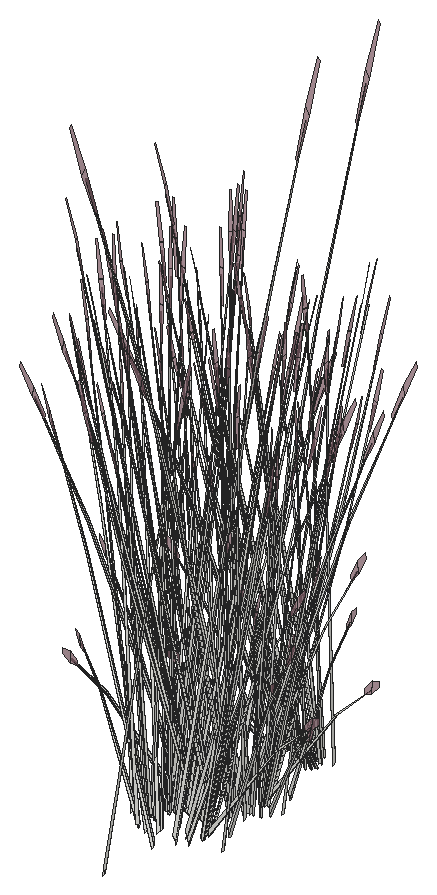
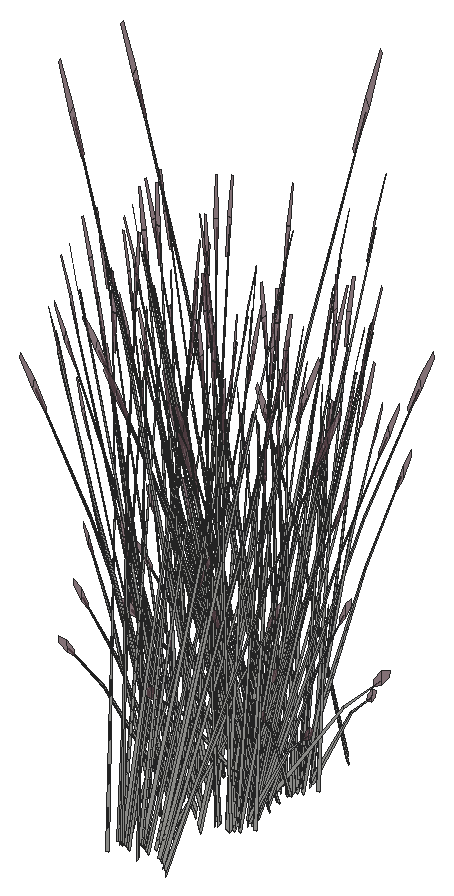
# SketchUp Ruby script. Lengths in inches.
U = 1.inch
M = Sketchup.active_model
def pt(a) = Geom::Point3d.new(a.map { |v| v * U })
def face(e, loops, mat)
  f = e.add_face(loops[0].map { |a| pt(a) })
  loops[1..].each { |l| e.add_face(l.map { |a| pt(a) }).erase! }
  f.material = f.back_material = mat if mat
  f
end
# faces: each face lists its corners as indices into pts; further lists are holes
def faces(e, pts, list, mat = nil) = list.each { |f| face(e, (f[0].is_a?(Array) ? f : [f]).map { |l| l.map { |i| pts[i] } }, mat) }
# xy, xz, yz: faces in a plane at the given z, y or x. An outline is a flat list of corners, or four numbers for a rectangle; further outlines are holes
def ring(l) = l.size == 4 ? [[l[0], l[1]], [l[2], l[1]], [l[2], l[3]], [l[0], l[3]]] : l.each_slice(2).to_a
def flat(e, list, mat, &to3) = list.each { |f| face(e, (f[0].is_a?(Array) ? f : [f]).map { |l| ring(l).map { |u, v| to3.(u, v) } }, mat) }
def xy(e, z, list, mat = nil) = flat(e, list, mat) { |x, y| [x, y, z] }
def xz(e, y, list, mat = nil) = flat(e, list, mat) { |x, z| [x, y, z] }
def yz(e, x, list, mat = nil) = flat(e, list, mat) { |y, z| [x, y, z] }
def lines(e, pts, list) = list.each { |a, b| e.add_line(pt(pts[a]), pt(pts[b])) }
# prism: a flat outline (further loops are holes) pulled along v
def prism(e, loops, v, mat = nil)
  f = face(e, loops, mat); d = Geom::Vector3d.new(v.map { |x| x * U })
  f.pushpull(f.normal.samedirection?(d) ? d.length : -d.length)
end
def box(e, o, s, mat = nil) = prism(e, [[o, [o[0] + s[0], o[1], o[2]], [o[0] + s[0], o[1] + s[1], o[2]], [o[0], o[1] + s[1], o[2]]]], [0, 0, s[2]], mat)
def at(x, y, z, deg = 0) = Geom::Transformation.translation(pt([x, y, z])) * Geom::Transformation.rotation(ORIGIN, Z_AXIS, deg.degrees)
def axes(o, x, y, z) = Geom::Transformation.new([*x, 0, *y, 0, *z, 0, *pt(o).to_a, 1])
def part(name) = M.definitions.add(name)
# library, detail: a bought-in or finely detailed component or shape, given as its bounding box
def library(name, o, s) = part(name).tap { |d| box(d.entities, o, s) }
def detail(e, o, s) = box(e.add_group.entities, o, s)
def put(e, d, t, mat = nil) = e.add_instance(d, t).tap { |i| i.material = mat if mat }
def group(e, t, mat = nil) = e.add_group.tap { |g| g.transformation = t; g.material = mat if mat }.entities
root = M.entities
M.materials.add("LightPink_Translucent").color = [144, 107, 117]
M.materials["LightPink_Translucent"].alpha = 0.75
c1 = part("blade")
p = [[2.15,0.21,22],[0,0.17,0],[0.09,0.45,0],[2.18,0.31,22],[2.29,0.31,22],[0.38,0.45,0],
  [2.48,0.24,33],[2.49,0.24,33],[2.48,0.22,33]]
faces(c1.entities,p,[[0,1,2,3],[4,5,2,3],[6,3,4,7],[8,0,3,6]])
c2 = part("seeds")
p = [[0.3,-0.1,1.38],[-0.01,-0.03,1.59],[-0.01,-0.03,0.03],[0.14,-0.07,-0.07],[0.29,-0.03,3],[0.15,0.01,3.11]]
faces(c2.entities,p,[[0,1,2,3],[1,0,4,5]],"LightPink_Translucent")
c3 = part("blade with seeds")
put(c3.entities,c1,at(0,0,0))
put(c3.entities,c2,axes([2.4,0.25,30.99],[1.5799,-0.05474,1.17369],[-0.12525,1.92788,0.29478],[-0.07173,-0.02425,1.56792]))
put(root,c3,axes([429.55,431.71,154.25],[-0.40102,0.2196,-0.10273],[-0.19707,-0.38974,-0.57019],[-0.05291,-0.16424,0.8664]))
put(root,c3,axes([430.38,432.21,154.25],[-0.45039,-0.02337,-0.10273],[0.01231,-0.44247,-0.57019],[0.03129,-0.17041,0.8664]))
put(root,c3,axes([427.89,424.64,152.84],[0.009,-0.24349,1.30391],[0.40497,0.12861,0.18019],[-0.03509,0.2595,0.61571]))
put(root,c3,axes([430.35,431.92,153.82],[0.27728,-0.24833,-0.29918],[0.26248,0.28355,0.38624],[0.03994,-0.14407,0.73904]))
put(root,c3,axes([429.54,431.54,154],[0.30197,-0.1603,0.05432],[0.1478,0.29231,0.42765],[-0.02916,-0.12885,0.65209]))
put(root,c3,axes([428.35,431.62,153.82],[-0.06329,-0.37991,-0.29918],[0.36182,-0.10032,0.38624],[-0.09718,-0.10887,0.73904]))
put(root,c3,axes([431.05,429.17,154],[0.15051,0.3216,0.05432],[-0.27447,0.15741,0.42765],[0.12099,-0.03106,0.65209]))
put(root,c3,axes([431.03,429.05,154],[-0.11578,0.43006,0.40553],[-0.38064,-0.14706,0.33437],[0.14969,-0.02584,0.83914]))
put(root,c3,axes([428.51,431.58,154],[0.18625,-0.29962,0.05432],[0.26523,0.17444,0.42765],[-0.08575,-0.09606,0.65209]))
put(root,c3,axes([428.14,428.33,152.82],[0.11649,-0.06823,1.49584],[0.04017,0.47639,0.11706],[-0.25231,0.06321,0.53462]))
put(root,c3,axes([427.57,432.17,153.27],[0.15222,0.08126,1.44779],[-0.31502,0.34091,0.11706],[-0.19634,-0.15379,0.61892]))
put(root,c3,axes([431.71,430.45,153.98],[-0.03706,-0.04129,1.49853],[0.08106,-0.44261,-0.1416],[0.14596,-0.02828,0.26519]))
put(root,c3,axes([428.31,431.93,153.95],[-0.40438,0.11212,-0.43168],[-0.07074,-0.4246,-0.33437],[-0.10862,-0.12168,0.82598]))
put(root,c3,axes([430.35,432.02,154],[0.29182,0.32181,0.40553],[-0.3099,0.27755,0.33437],[0.05383,-0.15098,0.83914]))
put(root,c3,axes([428.59,431.55,154.59],[-0.2735,0.45217,-0.11506],[-0.39608,-0.2605,-0.63862],[-0.13768,-0.12775,0.97037]))
put(root,c3,axes([430.46,432.05,154],[0.33677,0.02198,0.05432],[-0.00923,0.33185,0.42765],[0.03524,-0.12712,0.65209]))
put(root,c3,axes([426.89,428.65,153.98],[-0.06692,0.06124,1.47793],[0.00569,0.44742,-0.23373],[-0.15339,0.05818,0.11853]))
put(root,c3,axes([427.34,428.59,153.95],[-0.11102,0.42903,-0.43168],[-0.38064,-0.14706,-0.33437],[-0.15325,0.03934,0.82598]))
put(root,c3,axes([427.32,428.22,154.25],[0.20619,0.42709,-0.10273],[-0.36595,0.20988,-0.57019],[-0.15422,0.05635,0.8664]))
put(root,c3,axes([431.39,430.08,153.32],[-0.07843,-0.39649,-0.0295],[0.37072,-0.09115,-0.13375],[0.07742,0.02514,0.44114]))
put(root,c3,axes([430.43,430.07,154.25],[0.02194,-0.47967,-0.10273],[0.41546,0.01311,-0.57019],[0.16001,0.03332,0.8664]))
put(root,c3,axes([430.6875,432.77,153.95],[-0.10528,-0.43067,-0.43168],[0.39868,-0.07534,-0.33437],[0.11425,-0.11568,0.82598]))
put(root,c3,axes([427.54,431.42,153.98],[-0.08817,-0.00333,1.47793],[-0.28072,0.33293,-0.23373],[-0.14978,-0.06803,0.11853]))
put(root,c3,axes([430.875,433.08,154.25],[-0.37908,-0.26007,-0.10273],[0.21839,-0.37663,-0.57019],[0.1071,-0.13092,0.8664]))
put(root,c3,axes([429.31,434.5,152.81],[0.35414,0.19019,1.27785],[-0.34693,0.40974,0.50532],[-0.1554,-0.24285,1.07126]))
put(root,c3,axes([430.79,429.78,153.98],[0.08791,-0.00798,1.47793],[0.24113,-0.36643,-0.23373],[0.15637,0.04837,0.11853]))
put(root,c3,axes([431.81,432.96,153.98],[-0.05353,-0.00358,1.49853],[-0.22227,-0.38383,-0.1416],[0.08926,-0.1262,0.26519]))
put(root,c3,axes([427.27,429.42,154],[-0.10163,-0.43409,0.40553],[0.39868,-0.07534,0.33437],[-0.1175,0.10209,0.83914]))
put(root,c3,axes([427.19,429.34,154],[-0.28133,-0.19836,0.05432],[0.16379,-0.28248,0.42765],[-0.0902,0.09132,0.65209]))
put(root,c3,axes([427.32,428.8125,153.27],[0.14219,-0.09977,1.44779],[0.11971,0.461,0.11706],[-0.22323,0.10419,0.61892]))
put(root,c3,axes([430.98,432.8125,153.82],[0.35672,-0.06741,-0.29918],[0.09419,0.38534,0.38624],[0.10222,-0.1035,0.73904]))
put(root,c3,axes([427.63,432.17,154],[0.02064,-0.35866,0.05432],[0.3116,0.00983,0.42765],[-0.11936,-0.03753,0.65209]))
put(root,c3,axes([427.51,432.28,153.82],[-0.23317,-0.29531,-0.29918],[0.26625,-0.27955,0.38624],[-0.13527,-0.04253,0.73904]))
put(root,c3,axes([426.14,429.1,153.98],[0.0523,0.01265,1.49853],[0.16179,0.41674,-0.1416],[-0.10706,0.10938,0.26519]))
put(root,c3,axes([430.69,430.03,153.82],[0.23317,0.29531,-0.29918],[-0.26625,0.27955,0.38624],[0.13527,0.04253,0.73904]))
put(root,c3,axes([430.57,430.15,154],[-0.02064,0.35866,0.05432],[-0.3116,-0.00983,0.42765],[0.11936,0.03753,0.65209]))
put(root,c3,axes([427.23,429.5,153.82],[-0.35672,0.06741,-0.29918],[-0.09419,-0.38534,0.38624],[-0.10222,0.1035,0.73904]))
put(root,c3,axes([430.6,430.03,154],[-0.30217,0.31079,0.40553],[-0.2606,-0.33005,0.33437],[0.14177,0.05733,0.83914]))
put(root,c3,axes([431.01,432.98,154],[0.28133,0.19836,0.05432],[-0.16379,0.28248,0.42765],[0.0902,-0.09132,0.65209]))
put(root,c3,axes([430.93,432.9,154],[0.10163,0.43409,0.40553],[-0.39868,0.07534,0.33437],[0.1175,-0.10209,0.83914]))
put(root,c3,axes([432.01,433.42,153.98],[0.05687,-0.07184,1.47793],[-0.07279,-0.44069,-0.23373],[0.14268,-0.08356,0.11853]))
put(root,c3,axes([429.86,429.27,153.27],[-0.15222,-0.08126,1.44779],[0.31502,-0.34091,0.11706],[0.19634,0.15379,0.61892]))
put(root,c3,axes([427.2,431.7,153.98],[0.03038,0.04707,1.49853],[-0.14646,0.42312,-0.1416],[-0.14833,0.00306,0.26519]))
put(root,c3,axes([429.88,428.21,153.78],[-0.35411,-0.24507,1.16821],[0.37391,-0.38156,0.50405],[0.11425,0.22994,1.12919]))
put(root,c3,axes([427.33,429.24,154.25],[0.37908,0.26007,-0.10273],[-0.21839,0.37663,-0.57019],[-0.1071,0.13092,0.8664]))
put(root,c3,axes([427.625,432.58,153.95],[-0.29757,0.31243,-0.43168],[-0.2606,-0.33005,-0.33437],[-0.15119,-0.04754,0.82598]))
put(root,c3,axes([429.61,430.59,154.25],[0.2442,-0.40372,-0.10273],[0.35364,0.23259,-0.57019],[0.12293,0.11406,0.8664]))
put(root,c3,axes([427.84,429.125,153.27],[0.10236,-0.14492,1.44779],[0.25844,0.39118,0.11706],[-0.17726,0.17814,0.61892]))
put(root,c3,axes([427.52,429.55,153.95],[0.10528,0.43067,-0.43168],[-0.39868,0.07534,-0.33437],[-0.11425,0.11568,0.82598]))
put(root,c3,axes([427.78,432.25,154.25],[-0.02194,0.47967,-0.10273],[-0.41546,-0.01311,-0.57019],[-0.16001,-0.03332,0.8664]))
put(root,c3,axes([430.89,434.09,154.25],[-0.20619,-0.42709,-0.10273],[0.36595,-0.20988,-0.57019],[0.15422,-0.05635,0.8664]))
put(root,c3,axes([429.29,430.92,153.98],[0.00121,-0.0571,1.49853],[0.35119,-0.25193,-0.1416],[0.12199,0.08992,0.26519]))
put(root,c3,axes([430.87,433.72,153.95],[0.11102,-0.42903,-0.43168],[0.38064,0.14706,-0.33437],[0.15325,-0.03934,0.82598]))
put(root,c3,axes([427.75,430.27,154],[-0.33677,-0.02198,0.05432],[0.00923,-0.33185,0.42765],[-0.03524,0.12712,0.65209]))
put(root,c3,axes([427.25,432.91,153.27],[0.16998,-0.01068,1.44779],[-0.11276,0.46299,0.11706],[-0.24224,-0.02864,0.61892]))
put(root,c3,axes([427.85,430.3,154],[-0.29182,-0.32181,0.40553],[0.3099,-0.27755,0.33437],[-0.05383,0.15098,0.83914]))
put(root,c3,axes([429.9,430.39,153.95],[0.40438,-0.11212,-0.43168],[0.07074,0.4246,-0.33437],[0.10862,0.12168,0.82598]))
put(root,c3,axes([429.7,430.73,154],[-0.18625,0.29962,0.05432],[-0.26523,-0.17444,0.42765],[0.08575,0.09606,0.65209]))
put(root,c3,axes([429.78,430.65,154],[-0.4076,0.10824,0.40553],[-0.07074,-0.4246,0.33437],[0.09586,0.12514,0.83914]))
put(root,c3,axes([427.77,429.48,153.27],[0.0763,-0.16212,1.44779],[0.3201,0.3355,0.11706],[-0.1444,0.2091,0.61892]))
put(root,c3,axes([427.18,433.26,154],[0.11578,-0.43006,0.40553],[0.38064,0.14706,0.33437],[-0.14969,0.02584,0.83914]))
put(root,c3,axes([427.15,433.15,154],[-0.15051,-0.3216,0.05432],[0.27447,-0.15741,0.42765],[-0.12099,0.03106,0.65209]))
put(root,c3,axes([428.66,430.78,154],[-0.30197,0.1603,0.05432],[-0.1478,-0.29231,0.42765],[0.02916,0.12885,0.65209]))
put(root,c3,axes([427.85,430.39,153.82],[-0.27728,0.24833,-0.29918],[-0.26248,-0.28355,0.38624],[-0.03994,0.14407,0.73904]))
put(root,c3,axes([426.9,430.32,153.98],[-0.01019,0.09334,1.47793],[0.28908,0.3247,-0.23373],[-0.07568,0.15355,0.11853]))
put(root,c3,axes([427.82,430.11,154.56],[0.45039,0.02337,-0.11403],[-0.01231,0.44247,-0.63292],[-0.03129,0.17041,0.9617]))
put(root,c3,axes([428.66,430.6,154.25],[0.40102,-0.2196,-0.10273],[0.19707,0.38974,-0.57019],[0.05291,0.16424,0.8664]))
put(root,c3,axes([431.1,433.92,153.82],[0.34057,0.13158,-0.29918],[-0.09933,0.38387,0.38624],[0.13712,-0.0352,0.73904]))
put(root,c3,axes([427.1,433.31,153.82],[-0.34057,-0.13158,-0.29918],[0.09933,-0.38387,0.38624],[-0.13712,0.0352,0.73904]))
put(root,c3,axes([428.13,430.28,154.23],[0.29336,0.31691,-0.47917],[-0.3099,0.27755,-0.37115],[-0.04464,0.16102,0.91684]))
put(root,c3,axes([429,430.58,153.95],[0.40284,0.11824,-0.43168],[-0.13808,0.40538,-0.33437],[0.03694,0.16321,0.82598]))
put(root,c3,axes([429.23,429.75,153.27],[-0.09368,-0.15143,1.44779],[0.43286,-0.12749,0.11706],[0.09783,0.23774,0.61892]))
put(root,c3,axes([430.18,433.45,153.27],[-0.16998,0.01068,1.44779],[0.11276,-0.46299,0.11706],[0.24224,0.02864,0.61892]))
put(root,c3,axes([428.82,430.83,153.82],[-0.12355,0.36271,-0.29918],[-0.36044,-0.10579,0.38624],[0.03305,0.14603,0.73904]))
put(root,c3,axes([431.05,434.08,154],[0.15051,0.3216,0.05432],[-0.27447,0.15741,0.42765],[0.12099,-0.03106,0.65209]))
put(root,c3,axes([431.03,433.97,154],[-0.11578,0.43006,0.40553],[-0.38064,-0.14706,0.33437],[0.14969,-0.02584,0.83914]))
put(root,c3,axes([428.04,430.13,154.51],[-0.01066,0.43628,-0.66621],[-0.44902,-0.0293,0.0804],[-0.04739,0.18483,0.94242]))
put(root,c3,axes([426.87,431.28,153.98],[0.04649,-0.02848,1.49853],[0.38427,0.18941,-0.1416],[-0.00903,0.15771,0.26519]))
put(root,c3,axes([428.46,429.82,153.27],[-0.01003,-0.18103,1.44779],[0.43473,0.12009,0.11706],[-0.02689,0.25798,0.61892]))
put(root,c3,axes([428.14,433.25,152.82],[0.11649,-0.06823,1.49584],[0.04017,0.47639,0.11706],[-0.25231,0.06321,0.53462]))
put(root,c3,axes([428.5625,431.48,153.98],[0.05195,0.07595,1.47793],[0.41921,0.02984,-0.23373],[0.04216,0.1675,0.11853]))
put(root,c3,axes([431.71,435.36,153.98],[-0.03706,-0.04129,1.49853],[0.08106,-0.44261,-0.1416],[0.14596,-0.02828,0.26519]))
put(root,c3,axes([426.89,433.5625,153.98],[-0.06692,0.06124,1.47793],[0.00569,0.44742,-0.23373],[-0.15339,0.05818,0.11853]))
put(root,c3,axes([427.34,433.5,153.95],[-0.11102,0.42903,-0.43168],[-0.38064,-0.14706,-0.33437],[-0.15325,0.03934,0.82598]))
put(root,c3,axes([427.32,433.14,154.25],[0.20619,0.42709,-0.10273],[-0.36595,0.20988,-0.57019],[-0.15422,0.05635,0.8664]))
put(root,c3,axes([431.39,434.99,153.32],[-0.07843,-0.39649,-0.0295],[0.37072,-0.09115,-0.13375],[0.07742,0.02514,0.44114]))
put(root,c3,axes([428.2,438.95,153.27],[0.09368,0.15143,1.44779],[-0.43286,0.12749,0.11706],[-0.09783,-0.23774,0.61892]))
put(root,c3,axes([430.43,434.98,154.25],[0.02194,-0.47967,-0.10273],[0.41546,0.01311,-0.57019],[0.16001,0.03332,0.8664]))
put(root,c3,axes([428.91,437.95,153.98],[-0.06268,-0.06613,1.47793],[-0.4183,0.04193,-0.23373],[-0.06676,-0.15817,0.11853]))
put(root,c3,axes([427.89,430.75,152.84],[0.009,-0.24349,1.30391],[0.40497,0.12861,0.18019],[-0.03509,0.2595,0.61571]))
put(root,c3,axes([430.79,434.69,153.98],[0.08791,-0.00798,1.47793],[0.24113,-0.36643,-0.23373],[0.15637,0.04837,0.11853]))
put(root,c3,axes([427.27,434.33,154],[-0.10163,-0.43409,0.40553],[0.39868,-0.07534,0.33437],[-0.1175,0.10209,0.83914]))
put(root,c3,axes([427.19,434.25,154],[-0.28133,-0.19836,0.05432],[0.16379,-0.28248,0.42765],[-0.0902,0.09132,0.65209]))
put(root,c3,axes([427.32,433.73,153.27],[0.14219,-0.09977,1.44779],[0.11971,0.461,0.11706],[-0.22323,0.10419,0.61892]))
put(root,c3,axes([430.79,438.76,153.98],[-0.00396,-0.09387,1.47793],[-0.33411,-0.2713,-0.23373],[0.05166,-0.16446,0.11853]))
put(root,c3,axes([429.39,438.74,153.82],[0.12355,-0.36271,-0.29918],[0.36044,0.10579,0.38624],[-0.03305,-0.14603,0.73904]))
put(root,c3,axes([429.66,439.22,153.27],[-0.0763,0.16212,1.44779],[-0.3201,-0.3355,0.11706],[0.1444,-0.2091,0.61892]))
put(root,c3,axes([430.7,438.42,153.98],[-0.04162,0.03603,1.49853],[-0.40776,-0.12155,-0.1416],[-0.01476,-0.15722,0.26519]))
put(root,c3,axes([429.21,438.99,153.95],[-0.40284,-0.11824,-0.43168],[0.13808,-0.40538,-0.33437],[-0.03694,-0.16321,0.82598]))
put(root,c3,axes([430.08,439.29,153.95],[-0.29336,-0.31691,-0.43168],[0.3099,-0.27755,-0.33437],[0.04464,-0.16102,0.82598]))
put(root,c3,axes([428.49,437.73,153.98],[-0.00765,0.05653,1.49853],[-0.37706,0.20517,-0.1416],[-0.11096,-0.10488,0.26519]))
put(root,c3,axes([426.14,434.02,153.98],[0.0523,0.01265,1.49853],[0.16179,0.41674,-0.1416],[-0.10706,0.10938,0.26519]))
put(root,c3,axes([429.43,438.82,154],[0.4038,0.12331,0.40553],[-0.13808,0.40538,0.33437],[-0.02427,-0.15942,0.83914]))
put(root,c3,axes([430.69,434.95,153.82],[0.23317,0.29531,-0.29918],[-0.26625,0.27955,0.38624],[0.13527,0.04253,0.73904]))
put(root,c3,axes([429.55,438.97,154.25],[-0.40102,0.2196,-0.10273],[-0.19707,-0.38974,-0.57019],[-0.05291,-0.16424,0.8664]))
put(root,c3,axes([430.38,439.46,154.25],[-0.45039,-0.02337,-0.10273],[0.01231,-0.44247,-0.57019],[0.03129,-0.17041,0.8664]))
put(root,c3,axes([430.57,435.06,154],[-0.02064,0.35866,0.05432],[-0.3116,-0.00983,0.42765],[0.11936,0.03753,0.65209]))
put(root,c3,axes([430.35,439.18,153.82],[0.27728,-0.24833,-0.29918],[0.26248,0.28355,0.38624],[0.03994,-0.14407,0.73904]))
put(root,c3,axes([429.54,438.79,154],[0.30197,-0.1603,0.05432],[0.1478,0.29231,0.42765],[-0.02916,-0.12885,0.65209]))
put(root,c3,axes([427.23,434.42,153.82],[-0.35672,0.06741,-0.29918],[-0.09419,-0.38534,0.38624],[-0.10222,0.1035,0.73904]))
put(root,c3,axes([428.35,438.87,153.82],[-0.06329,-0.37991,-0.29918],[0.36182,-0.10032,0.38624],[-0.09718,-0.10887,0.73904]))
put(root,c3,axes([430.6,434.94,154],[-0.30217,0.31079,0.40553],[-0.2606,-0.33005,0.33437],[0.14177,0.05733,0.83914]))
put(root,c3,axes([428.51,438.84,154],[0.18625,-0.29962,0.05432],[0.26523,0.17444,0.42765],[-0.08575,-0.09606,0.65209]))
put(root,c3,axes([429.86,434.1875,153.27],[-0.15222,-0.08126,1.44779],[0.31502,-0.34091,0.11706],[0.19634,0.15379,0.61892]))
put(root,c3,axes([427.57,439.42,153.27],[0.15222,0.08126,1.44779],[-0.31502,0.34091,0.11706],[-0.19634,-0.15379,0.61892]))
put(root,c3,axes([429.88,433.12,153.78],[-0.35411,-0.24507,1.16821],[0.37391,-0.38156,0.50405],[0.11425,0.22994,1.12919]))
put(root,c3,axes([427.33,434.15,154.25],[0.37908,0.26007,-0.10273],[-0.21839,0.37663,-0.57019],[-0.1071,0.13092,0.8664]))
put(root,c3,axes([429.61,435.5,154.25],[0.2442,-0.40372,-0.10273],[0.35364,0.23259,-0.57019],[0.12293,0.11406,0.8664]))
put(root,c3,axes([428.31,439.18,153.95],[-0.40438,0.11212,-0.43168],[-0.07074,-0.4246,-0.33437],[-0.10862,-0.12168,0.82598]))
put(root,c3,axes([430.35,439.27,154],[0.29182,0.32181,0.40553],[-0.3099,0.27755,0.33437],[0.05383,-0.15098,0.83914]))
put(root,c3,axes([428.59,438.81,154.59],[-0.2735,0.45217,-0.11506],[-0.39608,-0.2605,-0.63862],[-0.13768,-0.12775,0.97037]))
put(root,c3,axes([430.46,439.3,154],[0.33677,0.02198,0.05432],[-0.00923,0.33185,0.42765],[0.03524,-0.12712,0.65209]))
put(root,c3,axes([427.84,434.04,153.27],[0.10236,-0.14492,1.44779],[0.25844,0.39118,0.11706],[-0.17726,0.17814,0.61892]))
put(root,c3,axes([427.52,434.46,153.95],[0.10528,0.43067,-0.43168],[-0.39868,0.07534,-0.33437],[-0.11425,0.11568,0.82598]))
put(root,c3,axes([430.6875,440.02,153.95],[-0.10528,-0.43067,-0.43168],[0.39868,-0.07534,-0.33437],[0.11425,-0.11568,0.82598]))
put(root,c3,axes([429.29,435.84,153.98],[0.00121,-0.0571,1.49853],[0.35119,-0.25193,-0.1416],[0.12199,0.08992,0.26519]))
put(root,c3,axes([427.75,435.18,154],[-0.33677,-0.02198,0.05432],[0.00923,-0.33185,0.42765],[-0.03524,0.12712,0.65209]))
put(root,c3,axes([427.85,435.21,154],[-0.29182,-0.32181,0.40553],[0.3099,-0.27755,0.33437],[-0.05383,0.15098,0.83914]))
put(root,c3,axes([429.9,435.3,153.95],[0.40438,-0.11212,-0.43168],[0.07074,0.4246,-0.33437],[0.10862,0.12168,0.82598]))
